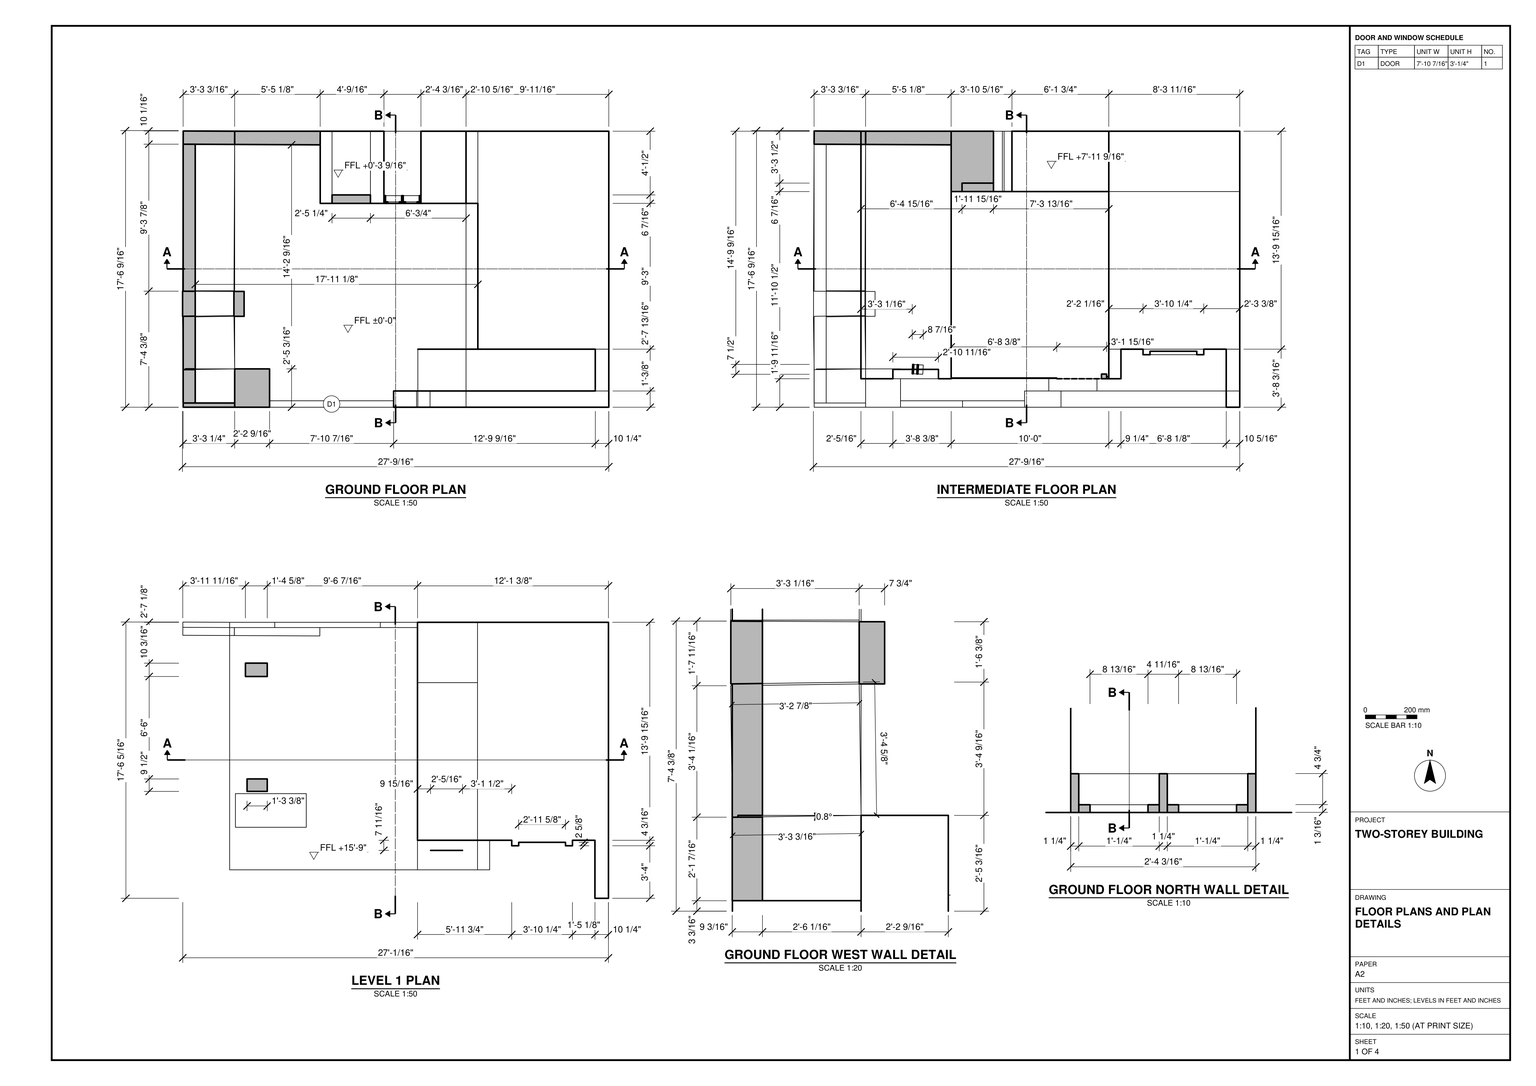
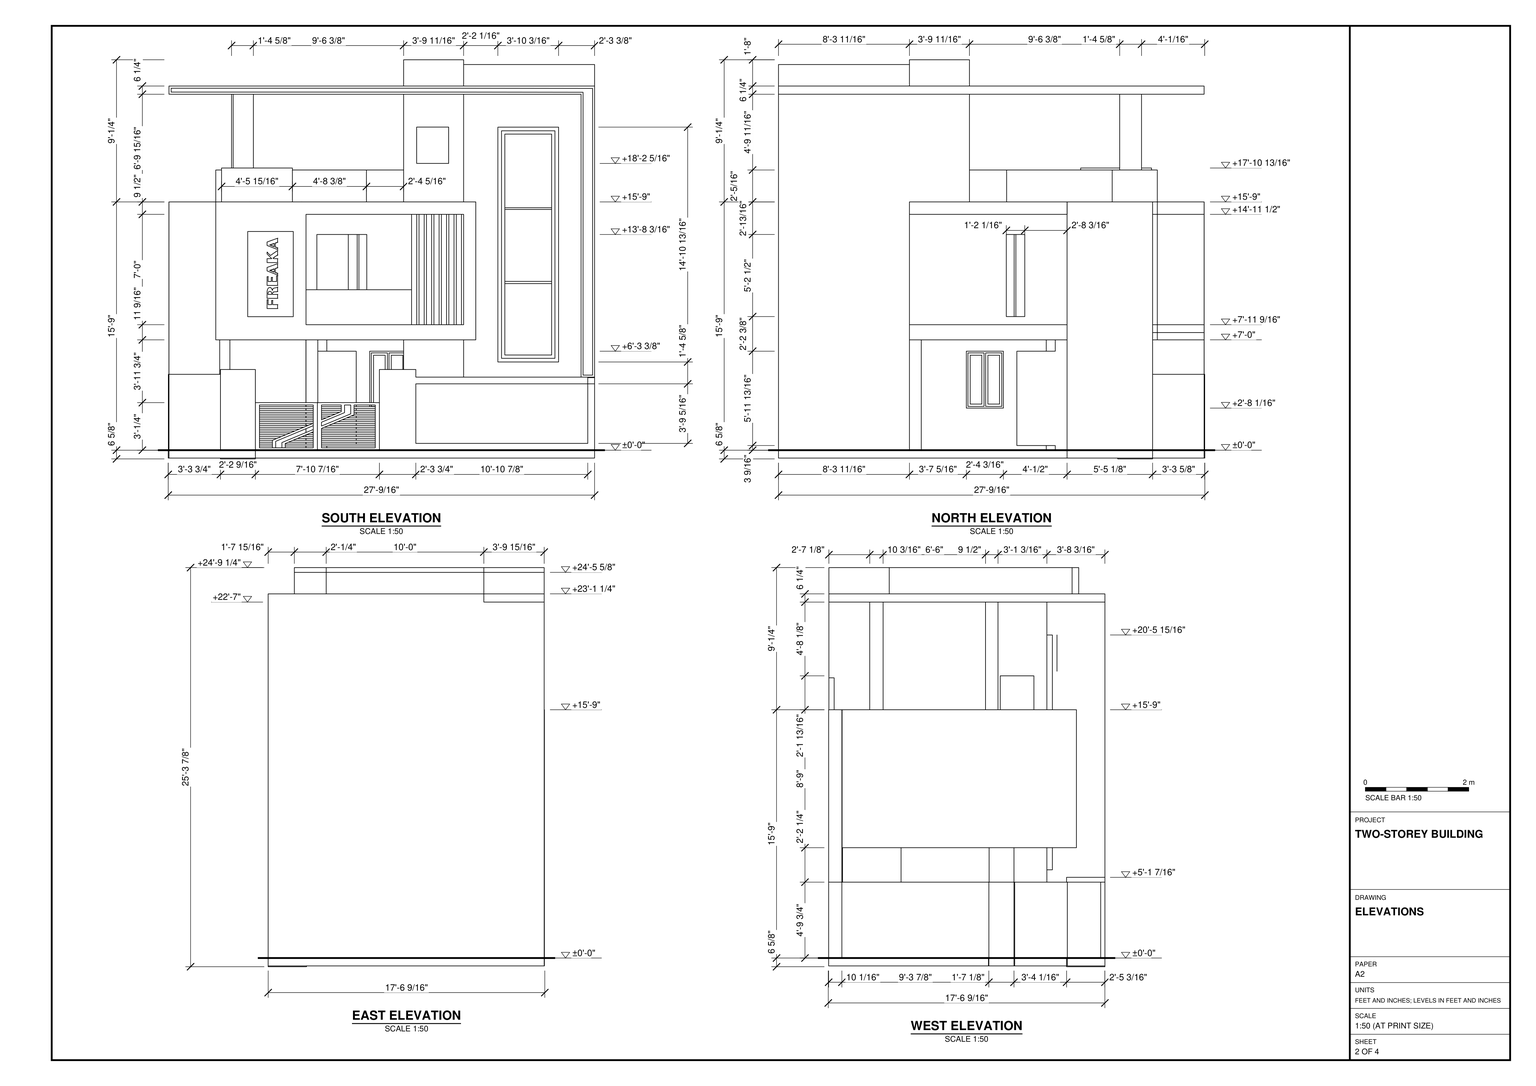
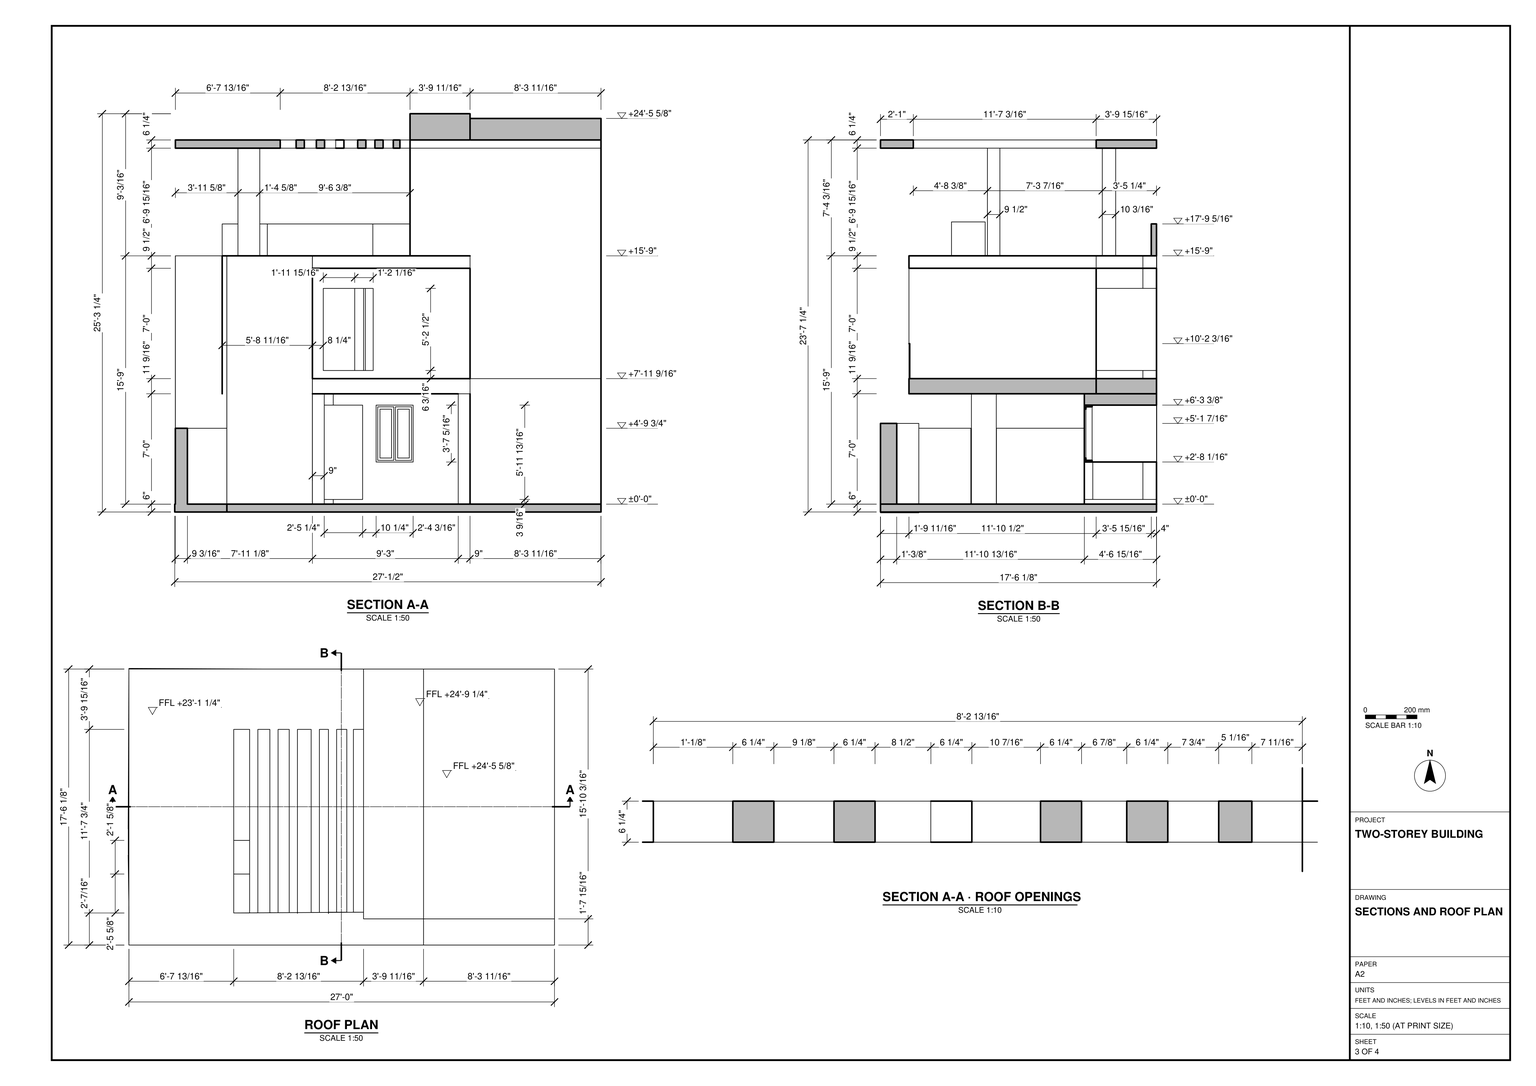
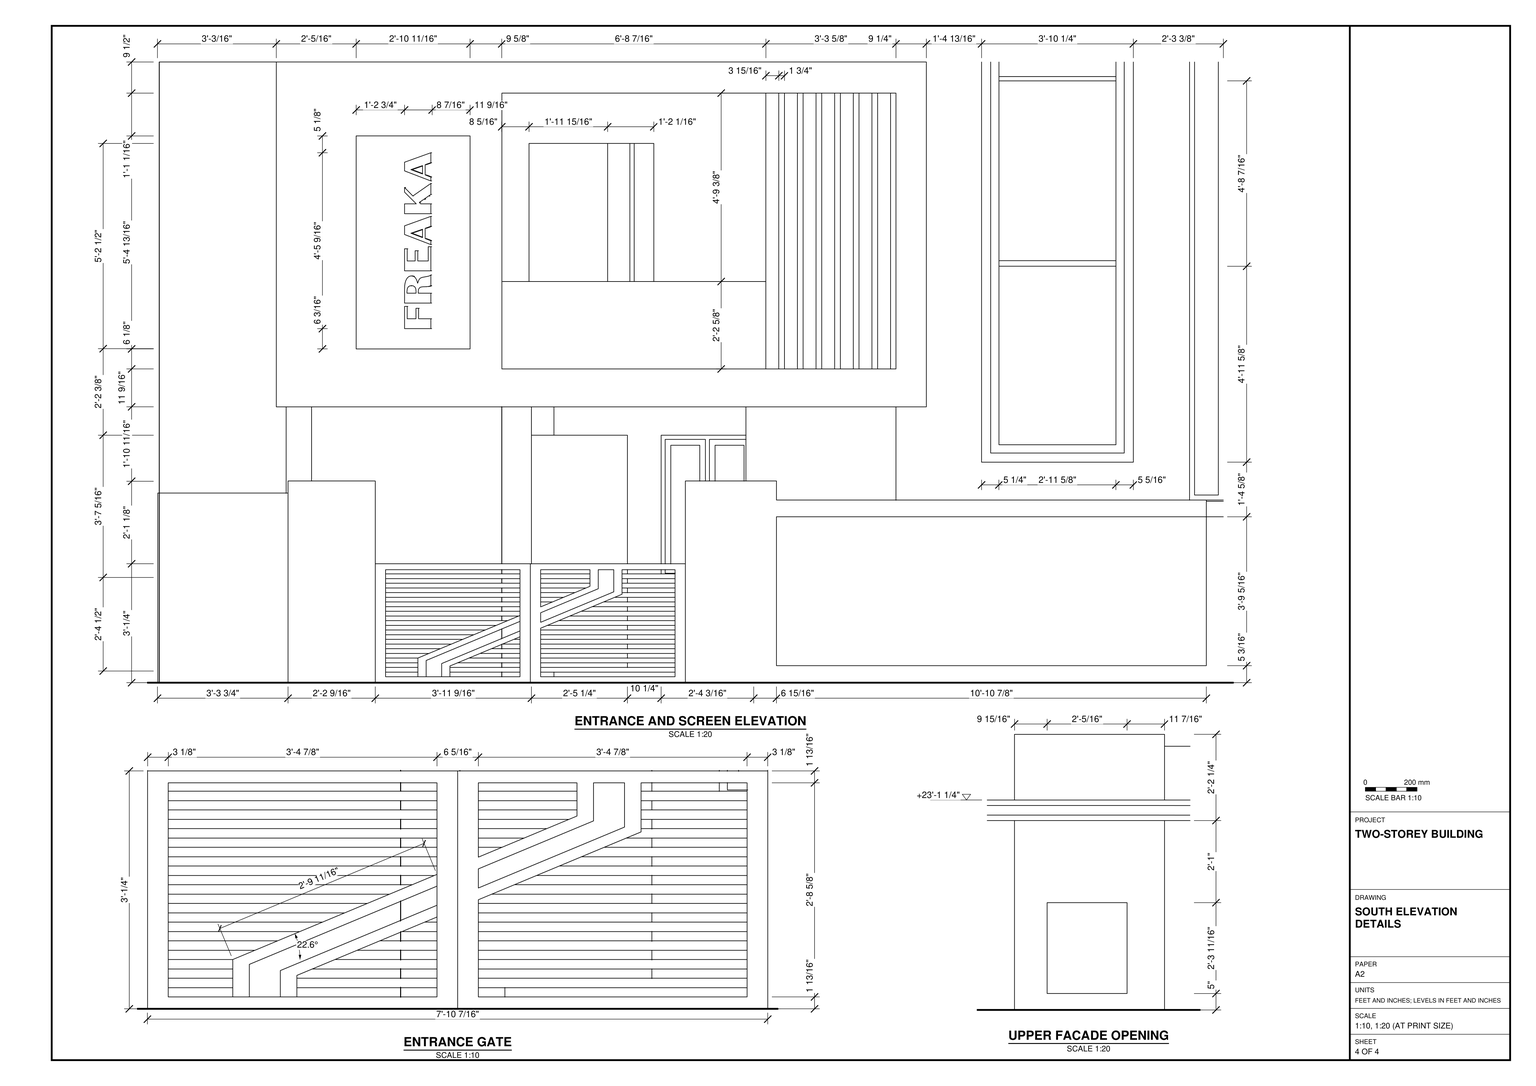
Build the two-storey building in SketchUp from task_files/diagram_01.pdf. Work in feet and inches. Set out the building with an overall width of 27'-9/16", depth of 17'-6 5/8" and height of 25'-3 7/8". Use ±0'-0" for the ground floor and +15'-9" for Level 1. Include the partial intermediate floor at +7'-11 9/16", following its outline in plan rather than extending it across the footprint.

Use the plans to locate the walls and openings, and the sections to set the wall and slab thicknesses as drawn. Follow the enlarged north and west wall details at ground level. On the south elevation, place the low entrance gate beneath the projecting rectangular frame. Include the lettered panel, recessed opening and vertical fins within the frame, and the tall framed panel to its right. Keep the east wall uninterrupted as shown. Model the upper supports, low parapets and stepped flat roof. Use the roof plan and section together to lay out the parallel roof openings.

Keep shell elements such as walls, slabs and roof sections, and each furniture or joinery piece shown, in separate groups or components. Use components for repeated parts. Decor and loose items may be any suitable library components. Save one SketchUp model as output_files/two_storey_building_with_a_slotted_flat_roof.skp.

# SketchUp Ruby script. Lengths in inches.
U = 1.inch
M = Sketchup.active_model
def pt(a) = Geom::Point3d.new(a.map { |v| v * U })
def face(e, loops, mat)
  f = e.add_face(loops[0].map { |a| pt(a) })
  loops[1..].each { |l| e.add_face(l.map { |a| pt(a) }).erase! }
  f.material = f.back_material = mat if mat
  f
end
# faces: each face lists its corners as indices into pts; further lists are holes
def faces(e, pts, list, mat = nil) = list.each { |f| face(e, (f[0].is_a?(Array) ? f : [f]).map { |l| l.map { |i| pts[i] } }, mat) }
# xy, xz, yz: faces in a plane at the given z, y or x. An outline is a flat list of corners, or four numbers for a rectangle; further outlines are holes
def ring(l) = l.size == 4 ? [[l[0], l[1]], [l[2], l[1]], [l[2], l[3]], [l[0], l[3]]] : l.each_slice(2).to_a
def flat(e, list, mat, &to3) = list.each { |f| face(e, (f[0].is_a?(Array) ? f : [f]).map { |l| ring(l).map { |u, v| to3.(u, v) } }, mat) }
def xy(e, z, list, mat = nil) = flat(e, list, mat) { |x, y| [x, y, z] }
def xz(e, y, list, mat = nil) = flat(e, list, mat) { |x, z| [x, y, z] }
def yz(e, x, list, mat = nil) = flat(e, list, mat) { |y, z| [x, y, z] }
def lines(e, pts, list) = list.each { |a, b| e.add_line(pt(pts[a]), pt(pts[b])) }
# prism: a flat outline (further loops are holes) pulled along v
def prism(e, loops, v, mat = nil)
  f = face(e, loops, mat); d = Geom::Vector3d.new(v.map { |x| x * U })
  f.pushpull(f.normal.samedirection?(d) ? d.length : -d.length)
end
def box(e, o, s, mat = nil) = prism(e, [[o, [o[0] + s[0], o[1], o[2]], [o[0] + s[0], o[1] + s[1], o[2]], [o[0], o[1] + s[1], o[2]]]], [0, 0, s[2]], mat)
def at(x, y, z, deg = 0) = Geom::Transformation.translation(pt([x, y, z])) * Geom::Transformation.rotation(ORIGIN, Z_AXIS, deg.degrees)
def axes(o, x, y, z) = Geom::Transformation.new([*x, 0, *y, 0, *z, 0, *pt(o).to_a, 1])
def part(name) = M.definitions.add(name)
# library, detail: a bought-in or finely detailed component or shape, given as its bounding box
def library(name, o, s) = part(name).tap { |d| box(d.entities, o, s) }
def detail(e, o, s) = box(e.add_group.entities, o, s)
def put(e, d, t, mat = nil) = e.add_instance(d, t).tap { |i| i.material = mat if mat }
def group(e, t, mat = nil) = e.add_group.tap { |g| g.transformation = t; g.material = mat if mat }.entities
root = M.entities
M.materials.add("Steve_Jacket1").color = [22, 22, 22]
M.materials.add("[Color I08]").color = [56, 24, 26]
M.materials.add("[Color K08]").color = [95, 0, 39]
M.materials.add("[Color L01]").color = [255, 248, 226]
M.materials.add("[Color M00]").color = [255, 255, 255]
M.materials.add("[Color M03]").color = [170, 170, 170]
M.materials.add("[Color M04]").color = [142, 142, 142]
M.materials["[Color M04]"].alpha = 0.39
M.materials.add("[Color M05]").color = [114, 114, 114]
M.materials.add("[Color M06]1").color = [86, 86, 86]
M.materials["[Color M06]1"].alpha = 0.91
M.materials.add("[Color M07]").color = [58, 51, 55]
M.materials.add("[Color M07]1").color = [58, 58, 58]
M.materials.add("[Color M09]").color = [0, 0, 0]
M.materials.add("[Translucent Glass Gray]").color = [132, 132, 132]
M.materials["[Translucent Glass Gray]"].alpha = 0.25
M.materials.add("[Translucent Glass Tinted]").color = [77, 201, 241]
M.materials["[Translucent Glass Tinted]"].alpha = 0.29
M.materials.add("[Wood Cherry Original]").color = [152, 86, 42]
M.materials["[Wood Cherry Original]"].alpha = 0.98
M.materials.add("[Wood Veneer 01]").color = [120, 70, 37]
c1 = part("Group\#8")
xy(c1.entities,0,[[0,0,19.69,1.18]],"[Wood Veneer 01]")
xy(c1.entities,2.76,[[2.76,0,16.93,1.18]],"[Wood Veneer 01]")
xy(c1.entities,60.24,[[2.76,0,16.93,1.18]],"[Wood Veneer 01]")
xy(c1.entities,62.99,[[0,0,19.69,1.18]],"[Wood Veneer 01]")
xz(c1.entities,0,[[2.76,2.76,16.93,60.24]],"[Translucent Glass Gray]")
xz(c1.entities,0,[[[0,0,19.69,62.99],[2.76,2.76,16.93,60.24]]],"[Wood Veneer 01]")
xz(c1.entities,1.18,[[[0,0,19.69,62.99],[2.76,2.76,16.93,60.24]]],"[Wood Veneer 01]")
yz(c1.entities,0,[[0,0,1.18,62.99]],"[Wood Veneer 01]")
yz(c1.entities,2.76,[[0,2.76,1.18,60.24]],"[Wood Veneer 01]")
yz(c1.entities,16.93,[[0,2.76,1.18,60.24]],"[Wood Veneer 01]")
yz(c1.entities,19.69,[[0,0,1.18,62.99]],"[Wood Veneer 01]")
c2 = part("pintu 2")
put(c2.entities,c1,at(-19.69,0,1.97))
g1 = group(c2.entities,at(-21.65,0,0))
prism(g1,[[[0,0,66.93],[0,0,0],[45.28,0,0],[45.28,0,66.93]],[[43.31,0,1.97],[23.62,0,1.97],[23.62,0,64.96],[43.31,0,64.96]],[[21.65,0,64.96],[21.65,0,1.97],[1.97,0,1.97],[1.97,0,64.96]]],[0,5.91,0],"[Wood Veneer 01]")
put(c2.entities,c1,at(1.97,0,1.97))
c3 = part("DOOR12")
g2 = group(c3.entities,at(114.73,28.14,-0.51))
g3 = group(g2,at(0,0,0))
box(g3,[0,0,0],[36,0.5,77.7])
c4 = library("Modern+Gate+1",[0,0,0],[118.11,1.97,78.74])
c5 = part("Freaka Letters")
g4 = group(c5.entities,at(1.09,0,0))
prism(g4,[[[0.31,0.04,0.58],[0.48,0.04,0],[0.42,0.04,0],[0.38,0.04,0.125],[0.2,0.04,0.125],[0.17,0.04,0],[0,0.04,0],[0.16,0.04,0.58]],[[0.22,0.04,0.18],[0.36,0.04,0.18],[0.29,0.04,0.44]]],[0,-0.04,0])
g5 = group(c5.entities,at(0.52,0,0))
prism(g5,[[[0.32,0.04,0.25],[0.1875,0.04,0],[0,0.04,0],[0.21,0.04,0.4],[0.07,0.04,0.58],[0.15,0.04,0.58],[0.35,0.04,0.32],[0.35,0.04,0.58],[0.52,0.04,0.58],[0.52,0.04,0],[0.35,0.04,0],[0.35,0.04,0.23]]],[0,-0.04,0])
g6 = group(c5.entities,at(1.61,0,0))
prism(g6,[[[0.41,0.04,0.58],[0.41,0.04,0],[0,0.04,0],[0,0.04,0.06],[0.24,0.04,0.06],[0.24,0.04,0.29],[0.07,0.04,0.29],[0.07,0.04,0.35],[0.24,0.04,0.35],[0.24,0.04,0.52],[0.04,0.04,0.52],[0.04,0.04,0.58]]],[0,-0.04,0])
g7 = group(c5.entities,at(0,0,0))
prism(g7,[[[0.31,0.04,0.58],[0.48,0.04,0],[0.42,0.04,0],[0.38,0.04,0.125],[0.2,0.04,0.125],[0.17,0.04,0],[0,0.04,0],[0.16,0.04,0.58]],[[0.22,0.04,0.18],[0.36,0.04,0.18],[0.29,0.04,0.44]]],[0,-0.04,0])
g8 = group(c5.entities,at(2.09,0,0))
prism(g8,[[[0.48,0,0],[0.48,0,0.58],[0.23,0,0.58],[0.18,0,0.58],[0.14,0,0.57],[0.11,0,0.56],[0.07,0,0.54],[0.05,0,0.52],[0.03,0,0.49],[0.02,0,0.46],[0.02,0,0.43],[0.02,0,0.38],[0.03,0,0.36],[0.05,0,0.34],[0.09,0,0.3125],[0.14,0,0.29],[0.09,0,0.27],[0.06,0,0.24],[0.04,0,0.2],[0.03,0,0.13],[0.02,0,0.05],[0.01,0,0.02],[0,0,0],[0.18,0,0],[0.2,0,0.05],[0.2,0,0.1],[0.2,0,0.14],[0.2,0,0.18],[0.21,0,0.22],[0.22,0,0.25],[0.25,0,0.27],[0.28,0,0.28],[0.3125,0,0.28],[0.3125,0,0]],[[0.3125,0,0.33],[0.28,0,0.33],[0.24,0,0.33],[0.21,0,0.35],[0.1875,0,0.38],[0.18,0,0.43],[0.1875,0,0.47],[0.21,0,0.5],[0.24,0,0.52],[0.28,0,0.53],[0.3125,0,0.53]]],[0,0.04,0])
g9 = group(c5.entities,at(2.625,0,0))
prism(g9,[[[0,0,0.58],[0,0,0.52],[0.21,0,0.52],[0.21,0,0.33],[0.03,0,0.33],[0.03,0,0.27],[0.21,0,0.27],[0.21,0,0],[0.38,0,0],[0.38,0,0.58]]],[0,0.04,0])
c6 = part("Group\#1")
xz(c6.entities,0,[[0,0,3.9375,84]])
xy(root,-6,[[0.582,0,0.582,28.625,2.261,28.649,39.761,29.1875,39.761,0],[39.761,0,39.761,69.219,46.937,69.219,46.937,88.156,39.761,88.156,39.761,210.125,104.878,210.125,104.878,0],[104.878,0,324.565,210.125],[0.582,28.625,0.582,28.649,0.008,68.657,0.32,68.661,39.187,69.219,39.761,29.1875,0.582,29.1875,0.582,28.649,2.261,28.649],[0.582,28.649,0.582,29.1875,39.761,29.1875,2.261,28.649],
  [39.761,29.1875,39.187,69.219,39.761,69.219],[0.32,68.661,0.3125,69.219,39.187,69.219],[0.1,69.219,0.1,88.34,39.187,88.156,39.761,88.156,39.761,69.219,39.187,69.219,39.179,69.779,0.3125,69.222,0.3125,69.219],[0.3125,69.219,0.3125,69.222,39.179,69.779,39.187,69.219],[39.761,69.219,46.937,88.156],
  [39.187,88.156,39.187,88.656,0.1,88.656,0.1,88.34,0,88.341,0.574,210.31,39.761,210.125,39.761,88.156],[39.187,88.156,0.1,88.34,0.1,88.656,39.187,88.656]])
xy(root,0,[[39.761,0,160.751,0,160.751,12.375,179.19,12.375,179.19,44.1875,215.878,44.1875,215.878,155.1875,104.878,155.1875,104.878,210.125,104.829,199.754,39.761,200.06],[160.751,0,178.211,12.375],[178.211,0,179.19,12.375],[179.19,0,188.489,12.375],[188.489,0,215.878,12.375],
  [215.878,0,324.565,12.375],[0.527,3.213,0.527,32.48,0.582,28.649,0.582,3.213],[0.582,3.213,0.582,28.625,2.261,28.649,9.73,28.649,9.73,3.213],[9.73,3.213,39.761,3.213,39.761,29.1875,9.73,28.757],[179.19,12.375,215.878,44.1875],
  [215.878,12.375,314.273,44.1875],[314.273,12.375,324.565,44.1875],[0.582,28.625,2.261,28.649,0.582,28.649],[0.582,28.649,2.261,29.1875],[2.261,28.649,9.73,28.649,9.73,28.757],
  [2.261,28.649,9.73,28.757,9.73,29.1875,2.261,29.1875],[9.73,28.757,39.761,29.1875,9.73,29.1875],[9.73,29.1875,39.761,29.1875,39.187,69.219,9.73,68.796],[39.761,29.1875,39.761,88.156,39.187,88.156,39.187,69.219],[0.527,32.48,0.527,68.664,0.32,68.661,0.008,68.657],
  [215.878,44.1875,224.878,155.1875],[224.878,44.1875,324.565,210.125],[0.32,68.661,0.527,68.664,0.519,69.225,0.3125,69.222,0.3125,69.219],[0.527,68.664,0.527,69.225,0.519,69.225],[0.527,68.664,0.527,69.225,9.722,69.357,9.73,68.796],
  [9.73,68.796,9.73,69.357,9.722,69.357],[9.73,68.796,39.187,69.219,39.179,69.779,9.73,69.357],[0.1,69.219,0.3125,69.219,0.3125,69.222,0.519,69.225,0.1,69.225],[39.187,69.219,39.187,88.156,9.73,88.295,9.73,69.357,39.179,69.779],[39.187,88.156,39.714,200.061,9.73,200.202,9.73,200.245,0.527,200.245,0,88.341,0.1,88.34,0.1,88.656,0.527,88.656,0.527,200.245,9.73,200.202,9.73,88.656,39.187,88.656],
  [39.187,88.156,39.187,88.656,9.73,88.656,9.73,88.295],[39.187,88.156,39.761,88.156,39.761,200.06,39.714,200.061],[0.1,88.338,0.527,88.338,0.1,88.34],[0.527,88.338,0.527,88.656,0.1,88.656,0.1,88.34],[104.878,155.1875,113.878,210.125],
  [113.878,155.1875,120.729,210.125],[120.729,155.1875,215.878,210.125],[215.878,155.1875,224.878,210.125],[39.761,200.06,39.761,210.125,39.714,200.061],[9.73,200.202,9.73,200.245,0.527,200.245],
  [39.761,210.125,104.878,210.125,0.576,210.616,0.574,210.31]])
xy(root,3.547,[[113.878,155.1875,143.104,210.125]])
xy(root,32.049,[[153.37,155.1875,181.558,210.125]])
xy(root,55.625,[[188.489,0,314.273,12.375]])
xy(root,57.75,[[0.582,0,39.761,3.213],[0.527,3.213,9.73,3.213,9.73,28.649,2.261,28.649,0.582,28.625,0.527,32.48],[0.582,28.625,2.261,28.649,2.261,29.1875,9.73,29.1875,9.73,68.796,9.722,69.357,0.527,69.225,0.519,69.225,0.527,68.664,0.527,32.48],[0.1,69.225,0.527,69.225,9.722,69.357,9.73,69.357,9.73,88.295,0.527,88.338,0.1,88.338],[9.73,88.295,9.73,200.202,0.527,200.245,0.527,88.338],
  [39.714,200.061,9.73,200.202,9.73,200.245,0.527,200.245,0.574,210.31,39.761,210.125],[9.73,200.202,0.527,200.245,9.73,200.245]])
xy(root,61.429,[[39.761,0,66.324,29.1875],[160.751,0,188.489,12.375]])
xy(root,67.155,[[250.942,40,297.161,44.1875]])
xy(root,72.452,[[256.239,40,291.864,42.625]])
xy(root,75.36,[[113.878,155.1875,143.104,210.125]])
xy(root,75.361,[[153.37,155.1875,181.558,210.125]])
xy(root,84,[[104.878,21.6875,113.878,155.1875],[113.878,21.6875,113.878,155.1875,215.878,155.1875,215.878,44.1875,179.19,44.1875,179.19,21.6875],[179.19,21.6875,215.878,44.1875],[215.878,21.6875,224.878,44.1875],[224.878,21.6875,234.128,44.1875],
  [104.878,155.1875,113.878,164.1875],[113.878,155.1875,120.729,164.1875],[120.729,155.1875,215.878,164.1875],[215.878,155.1875,224.878,164.1875],[104.878,164.1875,113.878,210.125],
  [113.878,164.1875,120.729,210.125],[120.729,164.1875,215.878,210.125],[215.878,164.1875,224.878,210.125]])
xy(root,95.542,[[104.878,21.6875,185.253,22.25],[185.253,21.6875,185.253,22.25,104.878,22.25,104.878,164.1875,224.878,164.1875,224.878,23.331,223.234,23.331,223.234,25.25,219.296,25.25,219.296,21.6875],[223.234,21.6875,224.878,23.331],[104.878,164.1875,224.878,210.125]])
xy(root,101.634,[[60.505,21.6875,95.193,28.8125]],"[Color I08]")
xy(root,101.722,[[137.08,164.1875,143.851,210.125],[143.851,164.1875,145.163,210.125],[145.163,164.1875,151.143,210.125]])
xy(root,122.167,[[104.878,21.6875,185.253,22.25]])
xy(root,164.222,[[137.08,164.1875,143.851,210.125],[143.851,164.1875,145.163,210.125],[145.163,164.1875,151.143,210.125]])
xy(root,166.509,[[60.505,21.6875,95.193,28.8125]])
xy(root,179.542,[[104.878,21.6875,219.296,21.6875,219.296,25.25,223.234,25.25,223.234,23.331,224.878,23.331,224.878,164.1875,104.878,164.1875],[219.296,21.6875,223.234,25.25],[223.234,21.6875,224.878,23.331],[104.878,164.1875,224.878,210.125]])
xy(root,189.022,[[179.19,21.6875,224.878,44.1875],[224.878,21.6875,234.128,44.1875],[179.19,44.1875,224.878,164.1875],[179.19,164.1875,224.878,210.125],[39.714,200.061,39.743,206.125,36.19,206.125,36.19,200.077],
  [36.19,200.077,36.19,206.142,0.556,206.31,0.527,200.245],[36.19,206.125,39.743,206.125,36.19,206.142],[39.743,206.125,39.761,210.125,36.19,210.125,36.19,206.142],[39.743,206.125,39.761,206.125,39.761,210.125],[39.761,206.125,70.534,210.125],
  [70.534,206.125,104.859,206.125,104.878,210.125,70.534,210.125],[104.859,206.125,104.878,206.125,104.878,210.125],[104.878,206.125,150.886,210.125],[150.886,206.125,179.19,210.125],[36.19,206.142,36.19,210.125,39.761,210.125,0.574,210.31,0.556,206.31]])
xy(root,189.022,[[104.829,199.754,104.859,206.125,39.761,206.125,39.761,200.06]],"[Color L01]")
xy(root,189.022,[[[36.19,21.6875,179.19,21.6875,179.19,206.125,104.859,206.125,104.829,199.754,39.761,200.06,39.761,206.125,39.743,206.125,39.714,200.061,36.19,200.077],[40.589,54.058,94.526,79.683],[48.207,168.855,64.817,179.043],[49.446,81.397,64.817,90.897]]],"[Color M05]")
xy(root,213.311,[[36.19,206.125,70.534,210.125],[70.534,206.125,150.886,210.125],[150.886,206.125,179.19,210.125]])
xy(root,214.835,[[40.589,54.058,94.526,79.683]],"[Wood Cherry Original]")
xy(root,240.64,[[256.239,40,291.864,42.625]])
xy(root,245.937,[[250.942,40,297.161,44.1875]])
xy(root,270.98,[[224.878,0,314.273,44.1875],[179.19,164.1875,324.565,210.125]])
xy(root,270.98,[[[0.574,0,0.574,210.125,179.19,210.125,179.19,164.1875,171.501,164.1875,171.501,25,179.19,25,179.19,44.1875,224.878,44.1875,224.878,0],[98.728,23.625,107.881,23.625,107.881,24.63,114.131,24.63,114.131,23.8125,122.62,23.8125,122.62,24.125,139.325,24.125,139.325,24.809,145.575,24.809,145.575,23.9375,152.455,23.9375,152.455,25,166.453,25,166.453,164.1875,158.705,164.1875,158.705,25,152.455,25,152.455,164.1875,145.575,164.1875,145.575,24.809,139.325,24.809,139.325,164.1875,128.87,164.1875,128.87,24.125,122.62,24.125,122.62,164.1875,114.131,164.1875,114.131,24.63,107.881,24.63,107.881,164.1875,98.728,164.1875,98.728,24.506,92.478,24.506,92.478,164.1875,80.381,164.1875,80.381,24.4375,92.478,24.4375,92.478,24.506,98.728,24.506],[48.207,168.855,64.817,179.043],[49.446,81.397,64.817,90.897]]],"[Color M03]")
xy(root,277.23,[[179.19,19.9375,224.878,164.1875],[224.878,19.9375,324.565,210.125],[80.381,24.4375,92.478,24.4375,92.478,24.506],[92.478,24.506,98.728,24.506,98.728,24.542],[158.705,24.883,166.453,24.927,166.453,25,158.705,25],
  [171.501,24.956,179.19,25,171.501,25],[179.19,164.1875,224.878,210.125]])
xy(root,277.23,[[0.574,0,224.878,0,224.878,19.9375,179.19,19.9375,179.19,25,171.501,24.956,166.453,24.927,158.705,24.883,152.455,24.848,145.575,24.809,139.325,24.773,128.87,24.714,122.62,24.678,114.131,24.63,107.881,24.594,98.728,24.542,98.728,24.506,92.478,24.506,92.478,24.4375,80.381,24.4375,80.381,164.1875,92.478,164.1875,92.478,24.506,98.728,24.542,98.728,164.1875,107.881,164.1875,107.881,24.63,114.131,24.63,114.131,164.1875,122.62,164.1875,122.62,24.678,128.87,24.714,128.87,164.1875,139.325,164.1875,139.325,24.809,145.575,24.809,145.575,164.1875,152.455,164.1875,152.455,25,158.705,25,158.705,164.1875,166.453,164.1875,166.453,24.927,171.501,24.956,171.501,164.1875,179.19,164.1875,179.19,210.125,0.574,210.125],[224.878,0,324.565,19.9375]],"[Color M06]1")
xy(root,293.605,[[224.878,19.9375,324.565,210.125]])
xy(root,297.23,[[179.19,19.9375,224.878,210.125]])
xz(root,0,[[66.324,-6,324.565,0],[315.795,57.147,323.043,57.147,323.043,275.431,223.217,275.569,2.235,275.569,2.235,272.64,223.217,272.64,315.795,272.502]])
xz(root,0,[[0.582,-6,66.324,-6,66.324,0,39.761,0,39.761,57.75,0.582,57.75],[188.489,5.185,319.38,50.523]],"[Color M00]")
xz(root,0,[[319.38,55.237,324.565,55.625],[[314.273,55.625,324.565,55.625,324.565,277.23,0.574,277.23,0.574,270.98,314.273,270.98],[315.795,57.147,315.795,272.502,223.217,272.64,2.235,272.64,2.235,275.569,223.217,275.569,323.043,275.431,323.043,57.147]]],"[Color M06]1")
xz(root,0,[[39.761,0,66.324,61.429],[[160.751,0,324.565,0,324.565,50.523,319.38,50.523,319.38,55.625,188.489,55.625,188.489,61.429,160.751,61.429],[188.489,5.185,319.38,50.523]]],"[Color M07]")
xz(root,0,[[319.38,50.523,324.565,55.237]],"[Color M07]1")
xz(root,3.213,[[0.527,0,0.582,57.75],[0.582,0,9.73,57.75],[9.73,0,39.761,57.75]])
xz(root,12.375,[[160.751,0,178.211,61.429],[178.211,0,188.489,61.429],[188.489,0,314.273,55.625]])
xz(root,19.9375,[[224.878,277.23,324.565,293.605]],"[Color M00]")
xz(root,19.9375,[[179.19,277.23,224.878,297.23]],"[Color M07]")
xz(root,21.6875,[[223.234,95.542,224.878,179.542]])
xz(root,21.6875,[[[36.19,84,234.128,189.022],[104.878,95.542,224.878,179.542],[60.505,101.634,95.193,166.509]]],"[Wood Veneer 01]")
xz(root,22.25,[[104.878,95.542,185.253,122.167]],"[Translucent Glass Tinted]")
xz(root,23.331,[[223.234,95.542,224.878,179.542]])
xz(root,24.4375,[[80.381,270.98,92.478,277.23]])
xz(root,24.506,[[92.478,270.98,98.728,277.23]])
xz(root,24.63,[[107.881,270.98,114.131,277.23]])
xz(root,24.809,[[139.325,270.98,145.575,277.23]])
xz(root,25,[[152.455,270.98,158.705,277.23],[158.705,270.98,166.453,277.23],[171.501,270.98,179.19,277.23]])
xz(root,25.25,[[219.296,95.542,223.234,179.542]])
xz(root,28.649,[[2.261,0,9.73,57.75]])
xz(root,28.8125,[[60.505,101.634,95.193,166.509]],"[Color I08]")
xz(root,29.1875,[[39.761,-6.633,66.324,61.429],[0.582,-6,39.761,0],[2.261,0,9.73,57.75]])
xz(root,36.48,[[189.129,218.314,213.473,245.982]],"Steve_Jacket1")
xz(root,40,[[[250.942,67.155,297.161,245.937],[253.718,69.932,294.384,243.16]]],"[Color M07]")
xz(root,40,[[[253.718,69.932,294.384,243.16],[256.239,72.452,291.864,240.64]]],"[Color M09]")
xz(root,42.625,[[256.239,126.827,291.864,128.515],[256.239,183.265,291.864,184.577]],"[Color M09]")
xz(root,42.625,[[256.239,72.452,291.864,126.827],[256.239,128.515,291.864,183.265],[256.239,184.577,291.864,240.64]],"[Translucent Glass Tinted]")
xz(root,44.1875,[[[224.878,0,314.273,0,314.273,270.98,224.878,270.98,224.878,189.022,234.128,189.022,234.128,84,224.878,84],[250.942,67.155,297.161,245.937]]],"[Color M00]")
xz(root,44.1875,[[179.19,0,224.878,84],[179.19,189.022,224.878,270.98]],"[Color M07]")
xz(root,54.058,[[40.589,189.022,94.526,214.835]],"[Wood Veneer 01]")
xz(root,69.219,[[39.187,-6,46.937,84]],"[Wood Veneer 01]")
xz(root,69.225,[[0.1,0,0.527,57.75],[0.519,0,0.527,57.75]])
xz(root,69.357,[[9.722,0,9.73,57.75]])
xz(root,79.683,[[40.589,189.022,94.526,214.835]])
xz(root,81.397,[[49.446,189.022,64.817,270.98]],"[Color M03]")
xz(root,88.156,[[39.187,-6,39.761,0],[39.761,-6,39.761,0,39.187,0,39.187,84,46.937,84,46.937,-6]])
xz(root,88.338,[[0.1,0,0.527,57.75]])
xz(root,88.656,[[0.1,-6,39.187,0]])
xz(root,90.897,[[49.446,189.022,64.817,270.98]],"[Color M04]")
xz(root,155.1875,[[104.878,0,113.878,0,113.878,3.547,143.104,3.547,143.104,75.36,113.878,75.36,113.878,84,104.878,84],[113.878,0,120.729,3.547],[215.878,0,224.878,84],[113.878,75.36,120.729,84]])
xz(root,155.1875,[[[120.729,0,215.878,0,215.878,84,120.729,84,120.729,75.36,143.104,75.36,143.104,3.547,120.729,3.547],[153.37,32.049,181.558,75.361]]],"[Color M00]")
xz(root,164.1875,[[104.878,84,224.878,95.542],[80.381,270.98,92.478,277.23],[98.728,270.98,107.881,277.23],[114.131,270.98,122.62,277.23],[128.87,270.98,139.325,277.23],
  [145.575,270.98,152.455,277.23],[158.705,270.98,166.453,277.23],[171.501,270.98,179.19,277.23]])
xz(root,164.1875,[[[104.878,95.542,224.878,179.542],[137.08,101.722,151.143,164.222]]],"[Color M00]")
xz(root,164.1875,[[143.851,101.722,145.163,164.222]],"[Color M09]")
xz(root,164.1875,[[137.08,101.722,143.851,164.222],[145.163,101.722,151.143,164.222]],"[Translucent Glass Tinted]")
xz(root,168.855,[[48.207,189.022,64.817,270.98]],"[Color M03]")
xz(root,179.043,[[48.207,189.022,64.817,270.98]],"[Color M04]")
xz(root,200.245,[[0.527,0,9.73,57.75]])
xz(root,206.125,[[36.19,189.022,70.534,213.311],[150.886,189.022,179.19,213.311]],"[Color M00]")
xz(root,206.125,[[70.534,189.022,150.886,213.311]],"[Translucent Glass Tinted]")
xz(root,210.125,[[39.761,-6,104.878,0],[104.878,-6,324.565,0],[39.761,0,104.878,189.022],[104.878,0,104.878,84,113.878,84,113.878,75.36,143.104,75.36,143.104,3.547,113.878,3.547,113.878,0],[113.878,0,120.729,3.547],
  [[120.729,0,120.729,3.547,143.104,3.547,143.104,75.36,120.729,75.36,120.729,84,215.878,84,215.878,0],[153.37,32.049,181.558,75.361]],[224.878,0,224.878,189.022,179.19,189.022,179.19,270.98,324.565,270.98,324.565,0],[215.878,0,224.878,84],[113.878,75.36,120.729,84],[36.19,84,39.761,89.542],
  [104.878,84,224.878,95.542],[36.19,89.542,39.761,95.542],[36.19,95.542,39.761,179.542],[[104.878,95.542,224.878,179.542],[137.08,101.722,151.143,164.222]],[36.19,179.542,39.761,189.022],
  [36.19,189.022,70.534,213.311],[70.534,189.022,150.886,213.311],[150.886,189.022,179.19,213.311],[0.574,270.98,324.565,277.23],[179.19,277.23,224.878,297.23],
  [224.878,277.23,324.565,293.605]])
yz(root,0.1,[[69.219,-6,88.34,0],[88.34,-6,88.656,0]])
yz(root,0.1,[[69.225,0,88.338,57.75]],"[Color M00]")
yz(root,0.527,[[3.213,0,68.664,57.75],[88.338,0,200.245,57.75]],"[Color M00]")
yz(root,0.574,[[0,270.98,210.125,277.23]])
yz(root,0.582,[[0,-6,0,57.75,3.213,57.75,3.213,0,28.625,0,28.625,-6],[28.625,-6,29.1875,0]])
yz(root,2.261,[[28.649,0,29.1875,57.75]])
yz(root,9.73,[[3.213,0,28.649,57.75],[29.1875,0,68.796,57.75],[69.357,0,88.295,57.75],[88.295,0,200.202,57.75],[200.202,0,200.245,57.75]])
yz(root,36.19,[[206.125,189.022,210.125,213.311]])
yz(root,36.19,[[21.6875,84,210.125,189.022]],"[Color M00]")
yz(root,39.187,[[88.156,-6,88.656,0]])
yz(root,39.187,[[69.219,0,88.156,84]],"[Wood Cherry Original]")
yz(root,39.761,[[0,-6.633,29.1875,-6],[29.1875,-6,88.156,0],[88.156,-6,210.125,0],[0,0,3.213,57.75],[3.213,0,3.213,57.75,0,57.75,0,61.429,29.1875,61.429,29.1875,0],
  [200.06,0,210.125,189.022]])
yz(root,40.589,[[54.058,189.022,79.683,214.835]],"[Wood Cherry Original]")
yz(root,46.937,[[69.219,-6,88.156,84]],"[Wood Veneer 01]")
yz(root,48.207,[[168.855,189.022,179.043,270.98]],"[Color M03]")
yz(root,49.446,[[81.397,189.022,90.897,270.98]],"[Color M03]")
yz(root,60.505,[[21.6875,101.634,28.8125,166.509]],"[Color I08]")
yz(root,64.817,[[168.855,189.022,179.043,270.98]],"[Color L01]")
yz(root,64.817,[[81.397,189.022,90.897,270.98]],"[Color M03]")
yz(root,66.324,[[0,-6.633,29.1875,61.429]],"[Color K08]")
yz(root,70.534,[[206.125,189.022,210.125,213.311]])
yz(root,80.381,[[24.4375,270.98,164.1875,277.23]])
yz(root,92.478,[[24.4375,270.98,24.506,277.23],[24.506,270.98,164.1875,277.23]])
yz(root,94.526,[[54.058,189.022,79.683,214.835]],"[Wood Cherry Original]")
yz(root,95.193,[[21.6875,101.634,28.8125,166.509]],"[Color I08]")
yz(root,98.728,[[24.506,270.98,164.1875,277.23]])
yz(root,104.878,[[155.1875,0,210.125,84],[164.1875,84,210.125,89.542],[164.1875,89.542,210.125,95.542],[21.6875,95.542,22.25,122.167],[22.25,95.542,164.1875,95.542,164.1875,179.542,21.6875,179.542,21.6875,122.167,22.25,122.167],
  [164.1875,95.542,210.125,179.542]])
yz(root,107.881,[[24.63,270.98,164.1875,277.23]])
yz(root,113.878,[[155.1875,0,210.125,3.547],[155.1875,75.36,210.125,84]])
yz(root,114.131,[[24.63,270.98,164.1875,277.23]])
yz(root,128.87,[[24.125,270.98,164.1875,277.23]])
yz(root,137.08,[[164.1875,101.722,210.125,164.222]])
yz(root,139.325,[[24.809,270.98,164.1875,277.23]])
yz(root,145.575,[[24.809,270.98,164.1875,277.23]])
yz(root,150.886,[[206.125,189.022,210.125,213.311]])
yz(root,151.143,[[164.1875,101.722,210.125,164.222]])
yz(root,152.455,[[23.9375,270.98,25,277.23],[25,270.98,164.1875,277.23]])
yz(root,153.37,[[155.1875,32.049,210.125,75.361]])
yz(root,158.705,[[25,270.98,164.1875,277.23]])
yz(root,160.751,[[0,0,12.375,61.429]])
yz(root,166.453,[[25,270.98,164.1875,277.23]])
yz(root,171.501,[[25,270.98,164.1875,277.23]])
yz(root,179.19,[[206.125,189.022,210.125,213.311],[19.9375,277.23,25,297.23],[25,277.23,164.1875,297.23],[164.1875,277.23,210.125,297.23]])
yz(root,179.19,[[44.1875,189.022,44.1875,270.98,25,270.98,25,277.23,164.1875,277.23,164.1875,270.98,210.125,270.98,210.125,213.311,206.125,213.311,206.125,189.022]],"[Color M00]")
yz(root,181.558,[[155.1875,32.049,210.125,75.361]])
yz(root,185.253,[[21.6875,95.542,22.25,122.167]])
yz(root,188.489,[[0,55.625,12.375,61.429]])
yz(root,215.878,[[155.1875,0,210.125,84]])
yz(root,219.296,[[21.6875,95.542,25.25,179.542]])
yz(root,223.234,[[21.6875,95.542,23.331,179.542],[23.331,95.542,25.25,179.542]])
yz(root,224.878,[[44.1875,0,155.1875,84],[164.1875,84,210.125,89.542],[164.1875,89.542,210.125,95.542],[21.6875,95.542,23.331,179.542],[23.331,95.542,164.1875,179.542],
  [164.1875,95.542,210.125,179.542],[164.1875,179.542,210.125,189.022],[19.9375,277.23,44.1875,293.605],[44.1875,277.23,164.1875,293.605],[164.1875,277.23,210.125,293.605],
  [19.9375,293.605,44.1875,297.23],[44.1875,293.605,164.1875,297.23],[164.1875,293.605,210.125,297.23]])
yz(root,234.128,[[21.6875,84,44.1875,95.542],[21.6875,95.542,44.1875,179.542],[21.6875,179.542,44.1875,189.022]],"[Wood Cherry Original]")
yz(root,250.942,[[40,67.155,44.1875,245.937]])
yz(root,256.239,[[40,72.452,42.625,128.515],[40,128.515,42.625,184.577],[40,184.577,42.625,240.64]])
yz(root,291.864,[[40,72.452,42.625,128.515],[40,128.515,42.625,184.577],[40,184.577,42.625,240.64]])
yz(root,297.161,[[40,67.155,44.1875,245.937]])
yz(root,314.273,[[12.375,0,12.375,55.625,0,55.625,0,270.98,44.1875,270.98,44.1875,0]],"[Color M00]")
yz(root,324.565,[[0,-6,210.125,0],[0,0,210.125,0,210.125,270.98,164.1875,270.98,164.1875,277.23,0,277.23],[164.1875,270.98,210.125,277.23],[19.9375,277.23,44.1875,293.605],[44.1875,277.23,164.1875,293.605],
  [164.1875,277.23,210.125,293.605]])
p = [[0.582,28.625,-6],[0.582,28.625,0],[0.582,28.649,0],[0.527,32.48,0],[0.008,68.657,0],[0.008,68.657,-6],
  [0.582,28.649,-6],[9.73,28.757,0],[2.261,28.649,0],[2.261,28.649,-6],[39.761,29.1875,-6],[39.761,29.1875,0],
  [39.187,69.219,-6],[39.187,69.219,0],[0.32,68.661,0],[0.32,68.661,-6],[9.73,68.796,0],[0.527,68.664,0],
  [0.3125,69.219,0],[0.3125,69.222,0],[0.3125,69.222,-6],[0.3125,69.219,-6],[39.179,69.779,0],[39.179,69.779,-6],
  [0.519,69.225,0],[0.527,69.225,0],[9.722,69.357,0],[9.73,69.357,0],[39.187,88.156,-6],[39.187,88.156,0],
  [9.73,88.295,0],[9.73,88.295,57.75],[0.527,88.338,57.75],[0.527,88.338,0],[0.1,88.34,0],[0.1,88.34,-6],
  [0,88.341,-6],[0,88.341,0],[0.574,210.31,-6],[0.527,200.245,0],[0.527,200.245,57.75],[0.574,210.31,57.75],
  [0.574,210.31,0],[39.761,210.125,0],[39.761,210.125,-6],[0.582,28.625,57.75],[2.261,28.649,57.75],[0.527,68.664,57.75],
  [0.519,69.225,57.75],[9.73,68.796,57.75],[9.722,69.357,57.75],[0.527,69.225,57.75],[39.761,200.06,0],[104.829,199.754,0],
  [104.829,199.754,189.022],[39.761,200.06,189.022],[104.878,210.125,0],[104.878,210.125,84],[104.878,210.125,89.542],[104.878,210.125,95.542],
  [104.878,210.125,179.542],[104.878,210.125,189.022],[104.859,206.125,189.022],[9.73,200.202,0],[39.714,200.061,0],[39.714,200.061,57.75],
  [9.73,200.202,57.75],[39.761,210.125,57.75],[39.714,200.061,189.022],[36.19,200.077,189.022],[0.527,200.245,189.022],[39.761,210.125,84],
  [39.761,210.125,89.542],[39.761,210.125,95.542],[39.761,210.125,179.542],[39.761,210.125,189.022],[39.743,206.125,189.022],[0.556,206.31,189.022],
  [0.574,210.31,189.022],[0.574,210.31,179.542],[0.574,210.31,95.542],[0.574,210.31,89.542],[0.574,210.31,84],[104.878,164.1875,189.022],
  [104.878,164.1875,179.542],[224.878,164.1875,95.542],[324.565,164.1875,95.542],[62.115,84.205,189.022],[62.115,84.205,189.085],[101.553,84.205,189.022],
  [101.553,84.205,189.085],[62.115,50.392,189.022],[62.115,50.392,189.085],[101.553,50.392,189.022],[101.553,50.392,189.085],[98.728,23.625,277.23],
  [98.728,23.625,270.98],[114.131,23.8125,277.23],[114.131,23.8125,270.98],[107.881,23.625,270.98],[107.881,23.625,277.23],[122.62,23.8125,270.98],
  [122.62,23.8125,277.23],[224.878,44.1875,270.98],[224.878,44.1875,277.23],[145.575,23.9375,277.23],[145.575,23.9375,270.98],[107.881,24.63,277.23],
  [107.881,24.594,277.23],[139.325,24.125,270.98],[139.325,24.125,277.23],[139.325,24.809,277.23],[139.325,24.773,277.23],[104.878,164.1875,89.542],
  [104.878,44.1875,89.542],[224.878,164.1875,89.542],[224.878,44.1875,89.542]]
faces(root,p,[[0,1,2,3,4,5,6],[7,8,1,0,9,10,11],[10,12,13,11],[4,14,15,5],[12,13,16,17,14,15],[15,14,18,19,20,21],[22,23,20,19,24,25,26,27],[13,12,23,22],
  [28,29,30,31,32,33,34,35],[36,35,34,37],[38,36,37,39,40,41,42],[43,44,38,42],[45,1,8,46],[17,47,48,24],[49,16,26,50],[26,25,51,50],
  [53,56,57,58,59,60,61,62,54],[63,64,65,66],[64,43,67,65],[39,63,66,40],[43,42,41,67],[65,68,69,70,40,66],[68,65,67,71,72,73,74,75,76],[40,70,77,78,79,80,81,82,41],
  [71,67,41,82],[72,71,82,81],[73,72,81,80],[74,73,80,79],[75,74,79,78]])
faces(root,p,[[52,53,54,55]],"[Color M00]")
lines(root,p,[[83,84],[85,86],[87,88],[89,90],[91,92],[93,94],[95,96],[97,98],[99,100],[101,102],[103,104],[105,106],
  [107,108],[109,110],[111,112],[113,114],[115,116]])
put(root,c2,axes([166.85,155.1875,32.05],[0.62258,0,0],[0,1,0],[0,0,0.64714]))
put(root,c3,axes([36.86,-198.23,102.13],[0.66493,0,0],[0,12.88,0],[0,0,0.8044]))
put(root,c3,axes([20.74,-207.23,4.02],[0.81185,0,0],[0,12.88,0],[0,0,0.92425]))
put(root,c4,axes([66.32,0,0],[0.79948,0,0],[0,2.49621,0],[0,0,0.46]))
put(root,c5,axes([83.65,32.13,161.39],[0,0,-17.82569],[-10.02133,-179.24469,0],[-13.77834,0.77033,0]))
put(root,c6,at(219.3,21.6875,95.54),"[Wood Veneer 01]")
put(root,c6,at(213.62,21.6875,95.54),"[Wood Veneer 01]")
put(root,c6,at(207.95,21.6875,95.54),"[Wood Veneer 01]")
put(root,c6,at(202.27,21.6875,95.54),"[Wood Veneer 01]")
put(root,c6,at(196.6,21.6875,95.54),"[Wood Veneer 01]")
put(root,c6,at(190.93,21.6875,95.54),"[Wood Veneer 01]")
put(root,c6,at(185.25,21.6875,95.54),"[Wood Veneer 01]")
g10 = group(root,at(188.49,0,5.18))
xz(g10,0,[[0,0,130.89,0,130.89,50.05,136.08,50.05,136.08,45.34,0,45.34]],"[Color M06]1")
